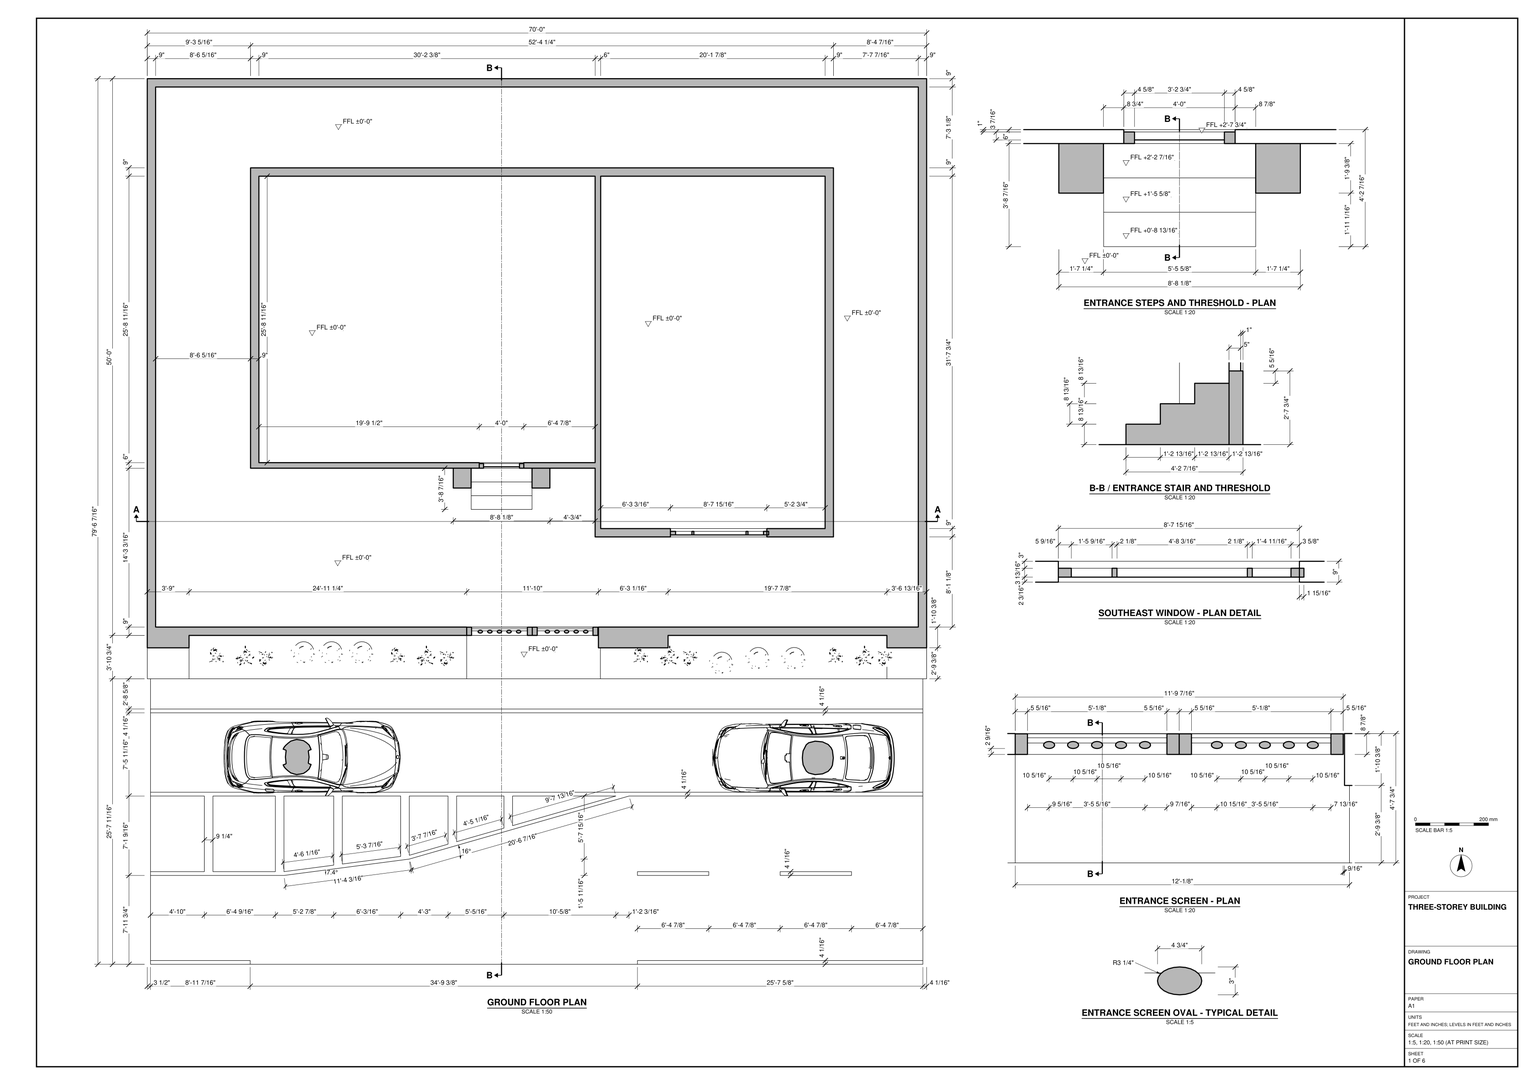
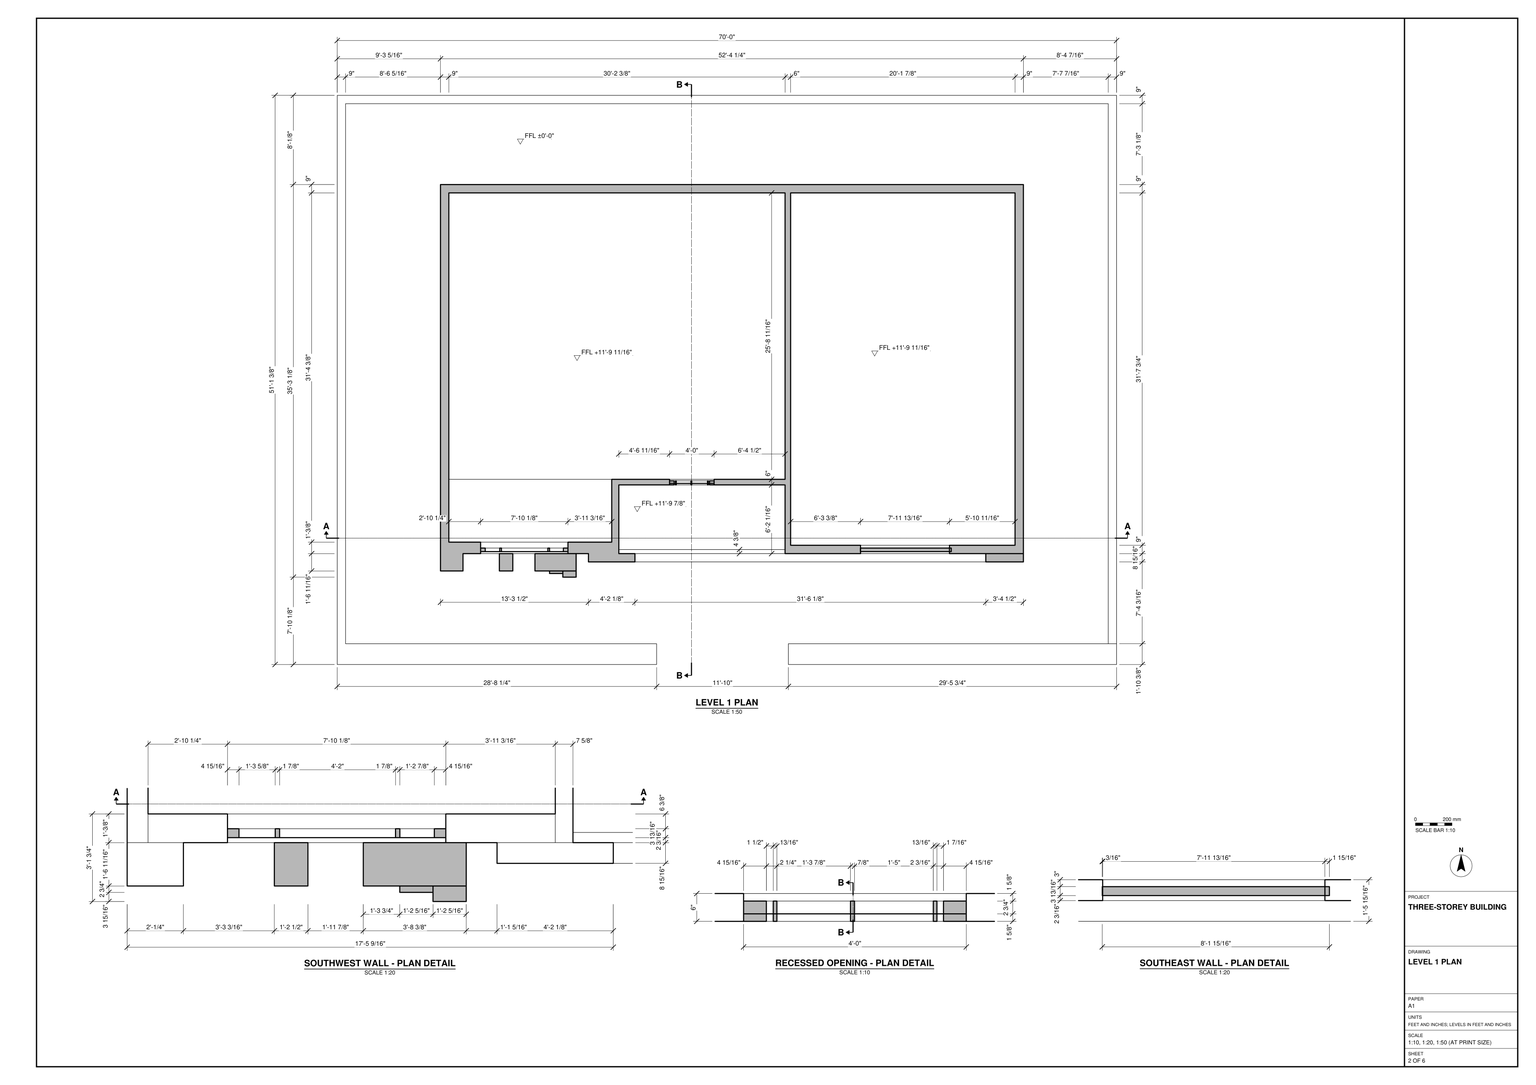
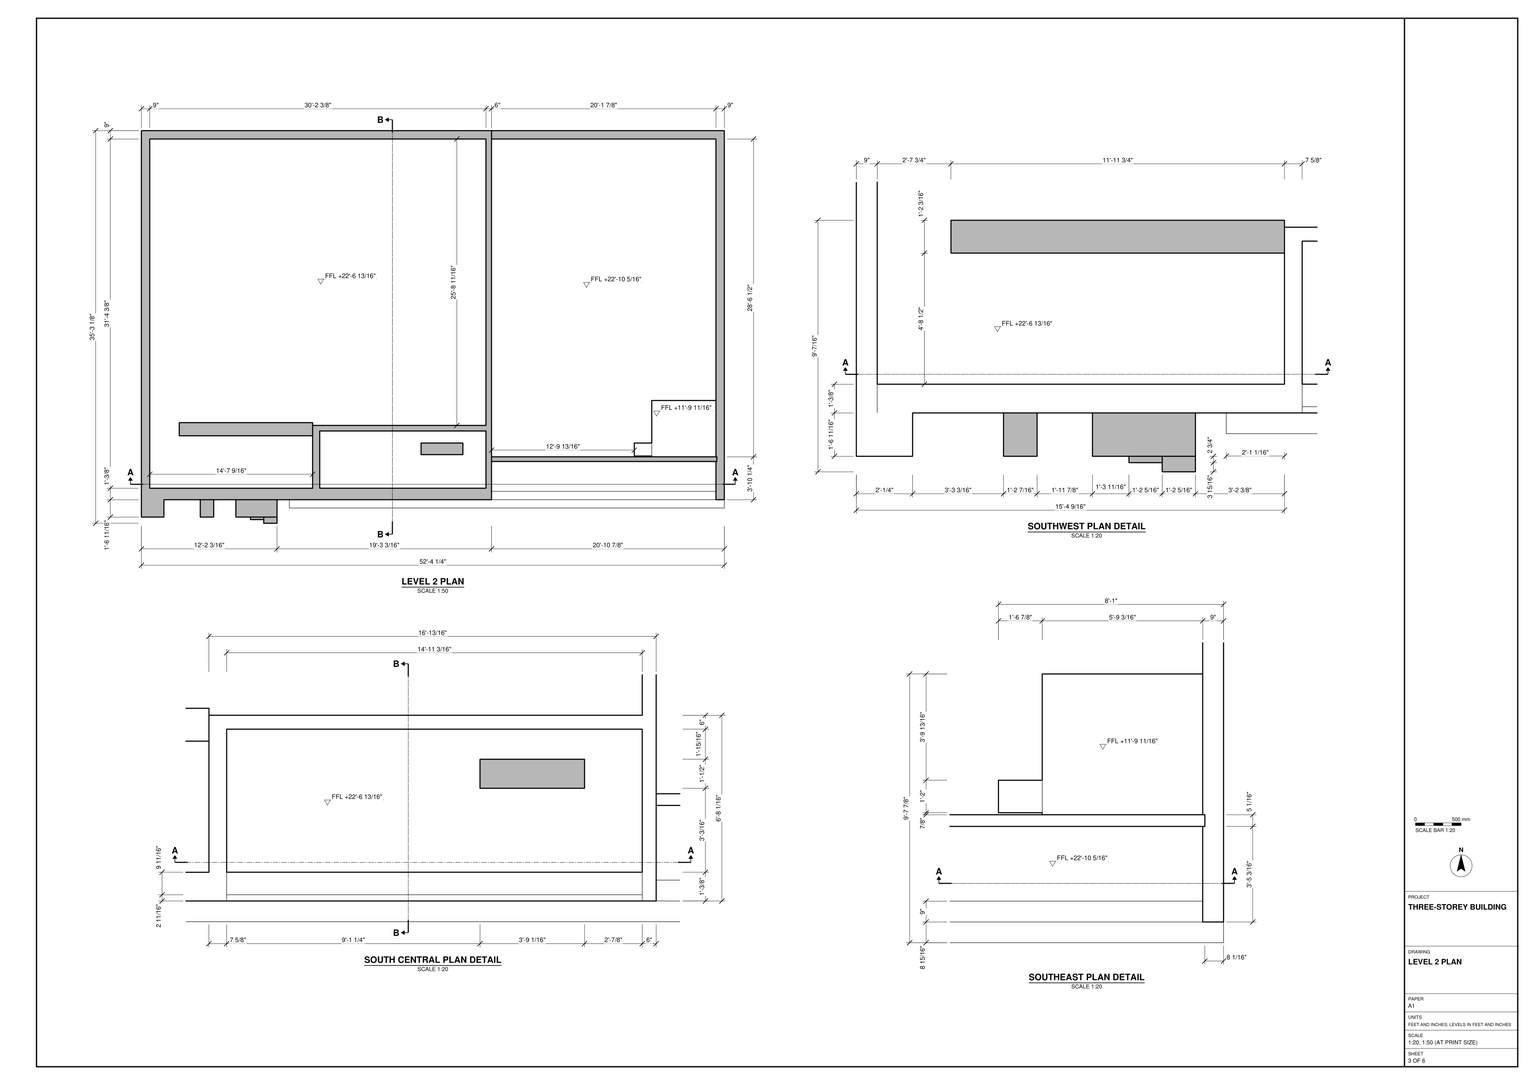
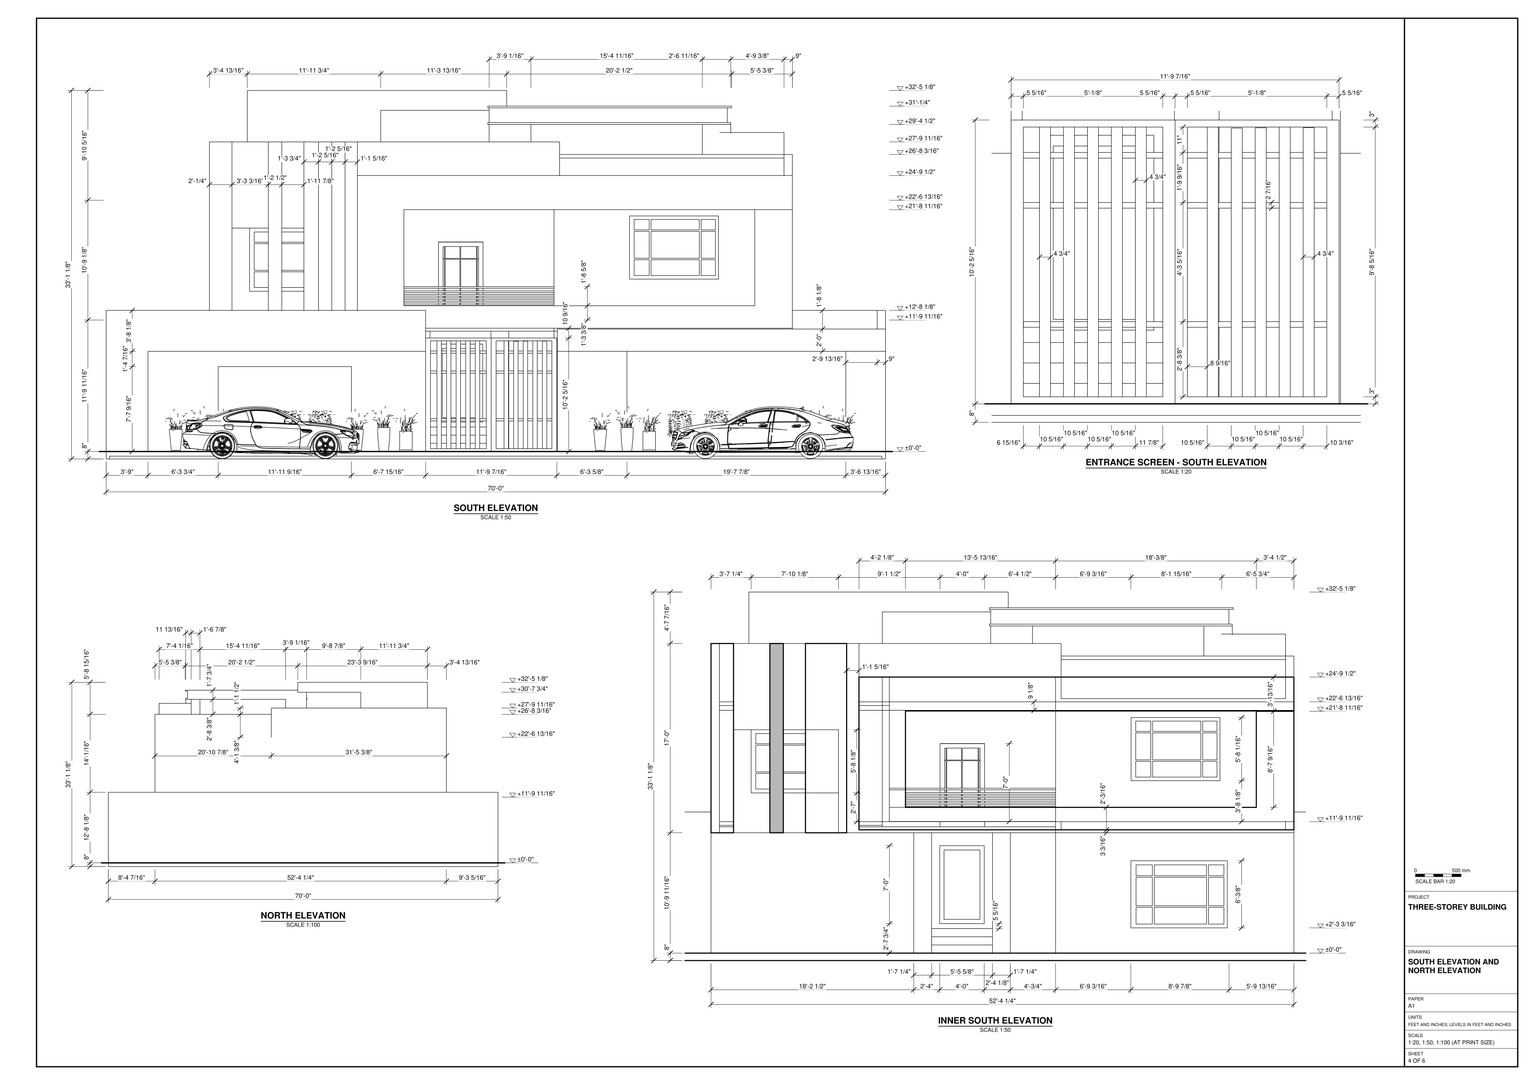
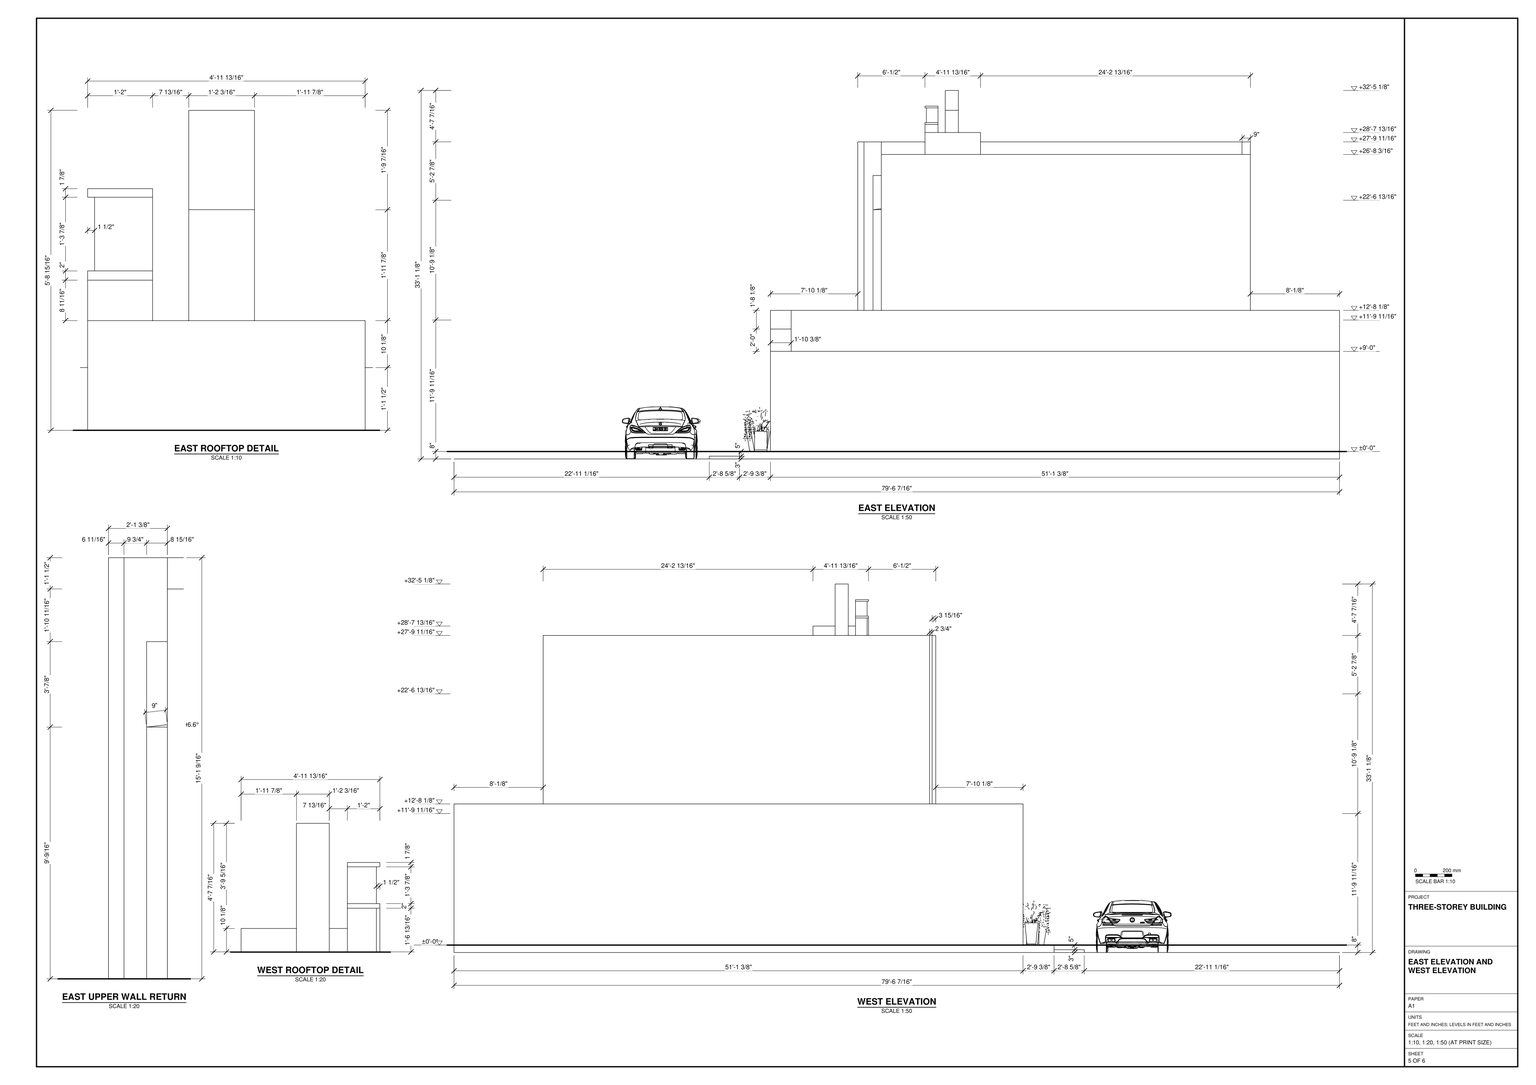
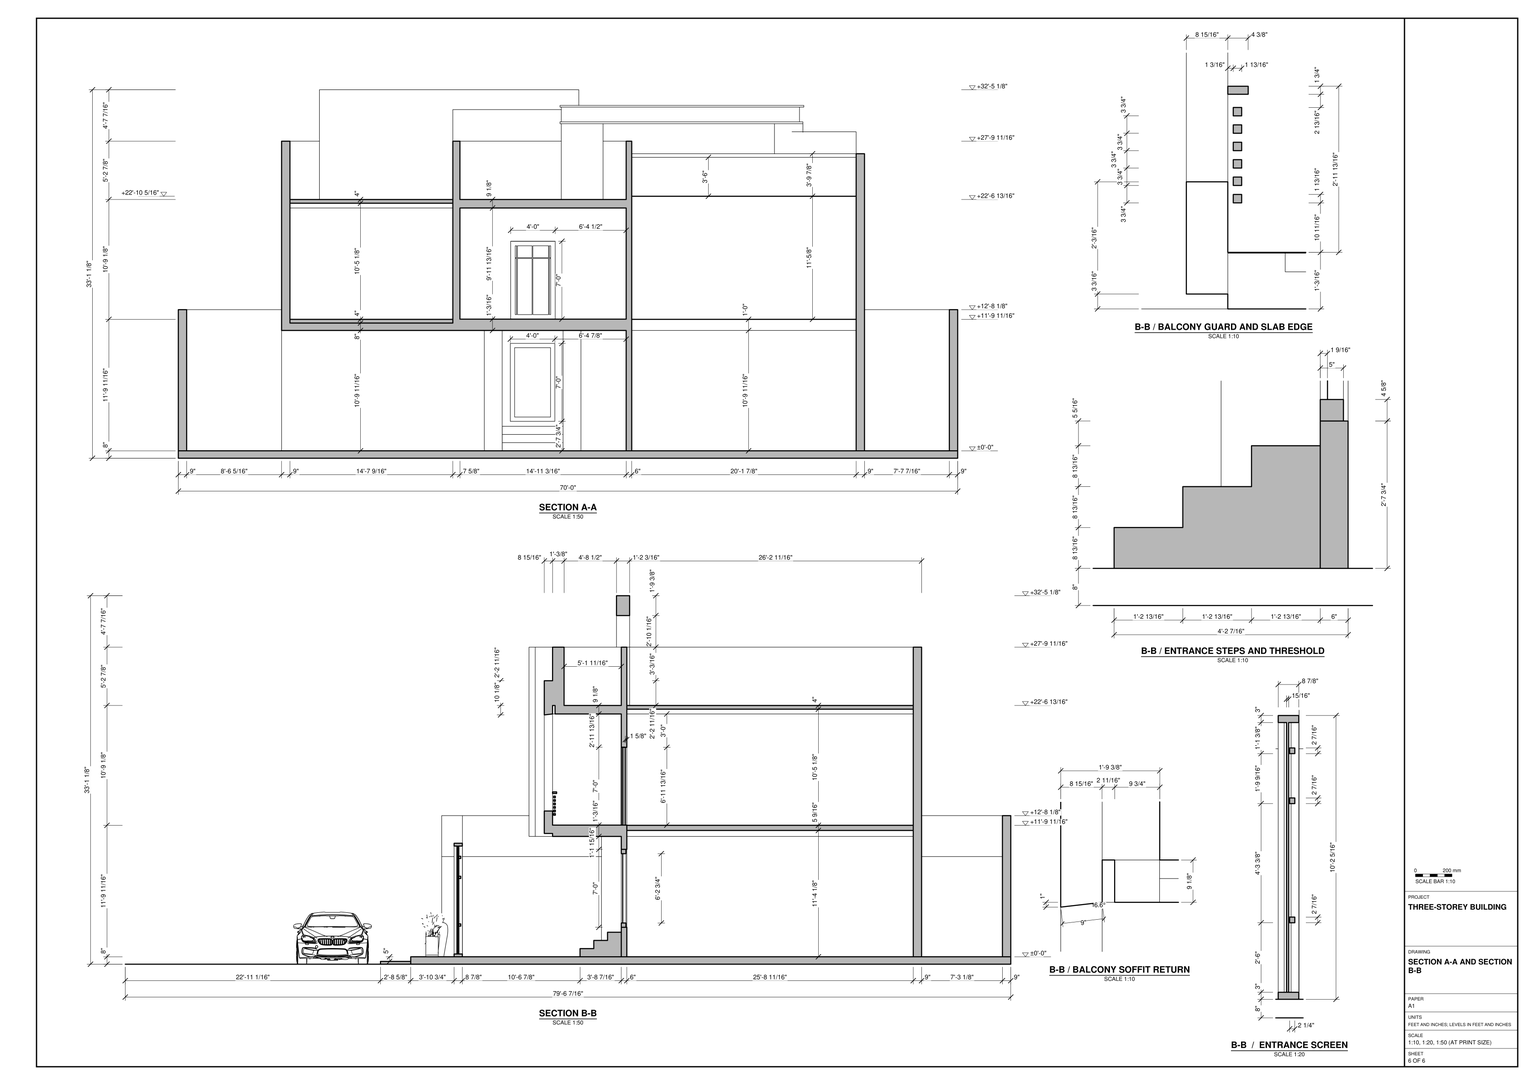
Build the three-storey building and its site in SketchUp from task_files/diagram_01.pdf. Work in feet and inches. Including the street frontage, the model measures 70'-0" across, 79'-6 7/16" from front to back and 33'-1 1/8" high. Set the principal floor levels to ±0'-0", +11'-9 11/16" and +22'-6 13/16". Follow the local changes in floor height shown on the plans.

Set the building back from the south boundary as drawn. Divide the shell into the wider west bay and narrower east bay, using the wall thicknesses shown. At ground level, extend the east bay forward of the west entrance wall. Model the entrance steps, threshold and door in the west bay and the framed window in the east bay. Use the upper-floor plans for the recessed central opening, the projecting portions of the southwest wall and the changes in slab outline at the southeast corner. Model the floor slabs and roof to the profiles shown rather than copying the ground-floor footprint upward.

Include the boundary walls, entrance screen, planting strips, two parked cars and street markings in their drawn positions. Planting, vehicles and other loose items may be suitable library components. Keep walls, slabs, roof and any individual furniture or joinery pieces in separate groups or components, and use components for repeated parts. Save one SketchUp model as output_files/three_storey_building_and_its_street_frontage.skp.

# SketchUp Ruby script. Lengths in inches.
U = 1.inch
M = Sketchup.active_model
def pt(a) = Geom::Point3d.new(a.map { |v| v * U })
def face(e, loops, mat)
  f = e.add_face(loops[0].map { |a| pt(a) })
  loops[1..].each { |l| e.add_face(l.map { |a| pt(a) }).erase! }
  f.material = f.back_material = mat if mat
  f
end
# faces: each face lists its corners as indices into pts; further lists are holes
def faces(e, pts, list, mat = nil) = list.each { |f| face(e, (f[0].is_a?(Array) ? f : [f]).map { |l| l.map { |i| pts[i] } }, mat) }
# xy, xz, yz: faces in a plane at the given z, y or x. An outline is a flat list of corners, or four numbers for a rectangle; further outlines are holes
def ring(l) = l.size == 4 ? [[l[0], l[1]], [l[2], l[1]], [l[2], l[3]], [l[0], l[3]]] : l.each_slice(2).to_a
def flat(e, list, mat, &to3) = list.each { |f| face(e, (f[0].is_a?(Array) ? f : [f]).map { |l| ring(l).map { |u, v| to3.(u, v) } }, mat) }
def xy(e, z, list, mat = nil) = flat(e, list, mat) { |x, y| [x, y, z] }
def xz(e, y, list, mat = nil) = flat(e, list, mat) { |x, z| [x, y, z] }
def yz(e, x, list, mat = nil) = flat(e, list, mat) { |y, z| [x, y, z] }
def lines(e, pts, list) = list.each { |a, b| e.add_line(pt(pts[a]), pt(pts[b])) }
# prism: a flat outline (further loops are holes) pulled along v
def prism(e, loops, v, mat = nil)
  f = face(e, loops, mat); d = Geom::Vector3d.new(v.map { |x| x * U })
  f.pushpull(f.normal.samedirection?(d) ? d.length : -d.length)
end
def box(e, o, s, mat = nil) = prism(e, [[o, [o[0] + s[0], o[1], o[2]], [o[0] + s[0], o[1] + s[1], o[2]], [o[0], o[1] + s[1], o[2]]]], [0, 0, s[2]], mat)
def at(x, y, z, deg = 0) = Geom::Transformation.translation(pt([x, y, z])) * Geom::Transformation.rotation(ORIGIN, Z_AXIS, deg.degrees)
def axes(o, x, y, z) = Geom::Transformation.new([*x, 0, *y, 0, *z, 0, *pt(o).to_a, 1])
def part(name) = M.definitions.add(name)
# library, detail: a bought-in or finely detailed component or shape, given as its bounding box
def library(name, o, s) = part(name).tap { |d| box(d.entities, o, s) }
def detail(e, o, s) = box(e.add_group.entities, o, s)
def put(e, d, t, mat = nil) = e.add_instance(d, t).tap { |i| i.material = mat if mat }
def group(e, t, mat = nil) = e.add_group.tap { |g| g.transformation = t; g.material = mat if mat }.entities
root = M.entities
M.materials.add("[Asphalt New]").color = [67, 60, 62]
M.materials.add("[Asphalt_New]").color = [67, 60, 62]
M.materials.add("[Color C08]").color = [102, 51, 0]
M.materials.add("[Color M00]").color = [255, 255, 255]
M.materials.add("[Color M06]").color = [86, 86, 86]
M.materials.add("[Color M08]").color = [58, 25, 30]
M.materials.add("[Color M09]").color = [74, 0, 0]
M.materials.add("[Color_000]").color = [255, 255, 255]
M.materials.add("[Color_D01]").color = [255, 191, 0]
M.materials.add("[Concrete_Form_4x8]").color = [167, 170, 168]
M.materials.add("[Granite Dark Gray]").color = [69, 68, 68]
M.materials.add("[Stone Vein Gray]").color = [166, 165, 165]
M.materials.add("[Translucent Glass Gray]").color = [128, 128, 128]
M.materials["[Translucent Glass Gray]"].alpha = 0.5
M.materials.add("[Wood Fence]").color = [142, 67, 30]
c1 = library("VASO VIETNAMITA",[-16.09,-10.89,0],[52.51,52.51,44.28])
c2 = part("Road w/ end turnlane")
xy(c2.entities,0,[[359.51,57.5,407.51,596]])
xy(c2.entities,0,[[[-39.49,57.5,-39.49,256.5,-45.49,256.5,-45.49,526.5,-39.49,526.5,-39.49,596,95.51,596,95.51,502.95,121.5,415.58,221.51,262.35,221.51,57.5],[95.51,107.25,101.51,157],[95.51,206.75,101.51,256.5]],[227.51,57.5,353.51,596],[221.51,271.54,174.5,343.5625,221.51,343.5625],[170.59,349.5625,149.04,382.57,221.51,382.57,221.51,349.5625],[145.125,388.57,127.5,415.58,221.51,415.58,221.51,388.57],
  [125.71,421.58,113.61,462.27,221.51,462.27,221.51,421.58],[111.83,468.27,101.51,502.95,221.51,502.95,221.51,468.27],[101.51,508.95,221.51,552.47],[101.51,558.47,221.51,596]],"[Asphalt_New]")
xy(c2.entities,0,[[353.51,57.5,359.51,596],[95.51,107.25,101.51,157],[95.51,206.75,101.51,256.5]],"[Color_000]")
xy(c2.entities,0,[[-45.49,57.5,-39.49,256.5],[[221.51,57.5,221.51,262.35,121.5,415.58,95.51,502.95,95.51,596,101.51,596,101.51,558.47,221.51,558.47,221.51,596,227.51,596,227.51,57.5],[101.51,508.95,221.51,552.47],[125.71,421.58,221.51,421.58,221.51,462.27,113.61,462.27],[111.83,468.27,221.51,468.27,221.51,502.95,101.51,502.95],[145.125,388.57,221.51,388.57,221.51,415.58,127.5,415.58],[170.59,349.5625,221.51,349.5625,221.51,382.57,149.04,382.57],[221.51,271.54,221.51,343.5625,174.5,343.5625]],[-45.49,526.5,-39.49,596]],"[Color_D01]")
xy(c2.entities,3,[[359.51,57.5,407.51,596]],"[Concrete_Form_4x8]")
xz(c2.entities,57.5,[[359.51,0,407.51,3]])
xz(c2.entities,596,[[359.51,0,407.51,3]],"[Concrete_Form_4x8]")
yz(c2.entities,359.51,[[57.5,0,596,3]],"[Concrete_Form_4x8]")
yz(c2.entities,407.51,[[57.5,0,596,3]],"[Concrete_Form_4x8]")
c3 = library("araç",[-7.9,-14.14,0],[84.07,190.26,56.29])
c4 = library("MERCEDES LIGHT",[-74.97,-97.73,0.18],[82.22,195.9,56.22])
c5 = part("Group\#1")
xy(c5.entities,0,[[0,0,100.125,6]],"[Color C08]")
xy(c5.entities,5.27,[[5.27,0,21.9,6],[23.9,0,77.06,6],[79.06,0,94.85,6]],"[Color C08]")
xy(c5.entities,26.63,[[5.27,0,21.9,6],[23.9,0,77.06,6],[79.06,0,94.85,6]],"[Color C08]")
xy(c5.entities,28.63,[[5.27,0,21.9,6],[23.9,0,77.06,6],[79.06,0,94.85,6]],"[Color C08]")
xy(c5.entities,65.04,[[5.27,0,21.9,6],[23.9,0,77.06,6],[79.06,0,94.85,6]],"[Color C08]")
xy(c5.entities,67.04,[[5.27,0,21.9,6],[23.9,0,77.06,6],[79.06,0,94.85,6]],"[Color C08]")
xy(c5.entities,80.98,[[5.27,0,21.9,6],[23.9,0,77.06,6],[79.06,0,94.85,6]],"[Color C08]")
xy(c5.entities,86.25,[[0,0,100.125,6]],"[Color C08]")
xz(c5.entities,0,[[[0,0,100.125,86.25],[23.9,28.63,77.06,65.04],[23.9,5.27,77.06,26.63],[23.9,67.04,77.06,80.98],[5.27,28.63,21.9,65.04],[79.06,28.63,94.85,65.04],[5.27,5.27,21.9,26.63],[79.06,5.27,94.85,26.63],[5.27,67.04,21.9,80.98],[79.06,67.04,94.85,80.98]]],"[Color C08]")
xz(c5.entities,0,[[5.27,5.27,21.9,26.63],[23.9,5.27,77.06,26.63],[79.06,5.27,94.85,26.63],[5.27,28.63,21.9,65.04],[23.9,28.63,77.06,65.04],
  [79.06,28.63,94.85,65.04],[5.27,67.04,21.9,80.98],[23.9,67.04,77.06,80.98],[79.06,67.04,94.85,80.98]],"[Translucent Glass Gray]")
xz(c5.entities,6,[[[0,0,100.125,86.25],[23.9,28.63,77.06,65.04],[23.9,5.27,77.06,26.63],[23.9,67.04,77.06,80.98],[5.27,28.63,21.9,65.04],[79.06,28.63,94.85,65.04],[5.27,5.27,21.9,26.63],[79.06,5.27,94.85,26.63],[5.27,67.04,21.9,80.98],[79.06,67.04,94.85,80.98]]],"[Color C08]")
yz(c5.entities,0,[[0,0,6,86.25]])
yz(c5.entities,5.27,[[0,5.27,6,26.63],[0,28.63,6,65.04],[0,67.04,6,80.98]],"[Color C08]")
yz(c5.entities,21.9,[[0,5.27,6,26.63],[0,28.63,6,65.04],[0,67.04,6,80.98]],"[Color C08]")
yz(c5.entities,23.9,[[0,5.27,6,26.63],[0,28.63,6,65.04],[0,67.04,6,80.98]],"[Color C08]")
yz(c5.entities,77.06,[[0,5.27,6,26.63],[0,28.63,6,65.04],[0,67.04,6,80.98]],"[Color C08]")
yz(c5.entities,79.06,[[0,5.27,6,26.63],[0,28.63,6,65.04],[0,67.04,6,80.98]],"[Color C08]")
yz(c5.entities,94.85,[[0,5.27,6,26.63],[0,28.63,6,65.04],[0,67.04,6,80.98]],"[Color C08]")
yz(c5.entities,100.125,[[0,0,6,86.25]],"[Color C08]")
c6 = library("Group\#2",[0,0,0],[48,4.375,84])
c7 = library("Group\#4",[0,0,0],[88.9375,8.875,134.4375])
c8 = library("Group\#6",[0,0,0],[79.77,27.28,49.07])
xy(root,0,[[0,307.71,840,954.46]])
xy(root,8,[[344.27,307.71,488.375,307.71,488.375,341.09,486.25,341.09,486.25,363.46,344.27,363.46],[0,341.09,0,954.46,840,954.46,840,341.09,797.19,341.09,797.19,354.46,561.29,354.46,561.29,341.09,486.25,341.09,486.25,363.46,831,363.46,831,945.46,9,945.46,9,363.46,344.27,363.46,344.27,354.46,45.03,354.46,45.03,341.09],[[9,363.46,831,945.46],[482.6875,460.59,482.6875,534.65,433.93,534.65,433.93,513.27,414.68,513.27,414.68,490.21,349.12,490.21,349.12,534.65,349.06,534.65,349.06,513.27,329.81,513.27,329.81,534.65,111.3125,534.65,111.3125,858.34,739.5625,858.34,739.5625,460.59]],[[482.6875,460.59,482.6875,534.65,111.3125,534.65,111.3125,858.34,739.5625,858.34,739.5625,460.59],[120.3125,540.65,482.6875,849.34],[488.6875,469.59,730.5625,849.34]],[488.6875,469.59,730.5625,849.34],
  [349.12,490.21,414.68,505.02],[349.12,505.02,414.68,534.65],[120.3125,540.65,482.6875,849.34]])
xy(root,8,[[0,307.71,45.03,341.09],[45.03,307.71,344.27,354.46],[488.375,307.71,797.19,307.71,797.19,354.46,561.29,354.46,561.29,341.09,488.375,341.09],[797.19,307.71,840,341.09]],"[Stone Vein Gray]")
xy(root,16.8125,[[349.12,490.21,414.68,505.02]])
xy(root,25.625,[[349.12,505.02,414.68,519.84]])
xy(root,34.4375,[[349.12,519.84,414.68,534.65]])
xy(root,35.21,[[563.85,460.59,667.79,469.59]])
xy(root,39.77,[[357.8125,534.65,405.8125,540.65]])
xy(root,107.58,[[563.85,460.59,667.79,469.59]])
xy(root,116,[[45.03,341.09,344.27,354.46],[486.25,341.09,486.25,363.46,840,363.46,840,341.09,797.19,341.09,797.19,354.46,561.29,354.46,561.29,341.09],[561.29,341.09,797.19,354.46]])
xy(root,123.77,[[357.8125,534.65,405.8125,540.65]])
xy(root,137.6875,[[243.17,435.21,257.49,441.9],[228.85,439.15,243.17,441.9],[111.3125,441.9,135.57,460.59],[174.77,441.9,189.24,460.59],[213.12,441.9,257.49,460.59],
  [111.3125,460.59,329.81,534.65],[329.81,460.59,349.06,513.27],[349.06,460.59,414.68,534.65],[414.68,460.59,433.93,513.27],[433.93,460.59,482.6875,534.65],
  [329.81,513.27,349.06,534.65],[414.68,513.27,433.93,534.65]])
xy(root,140,[[486.25,341.09,840,363.46]])
xy(root,140.9,[[270.78,451.65,739.5625,460.59]],"[Granite Dark Gray]")
xy(root,144.125,[[120.3125,540.65,482.6875,849.34]])
xy(root,145.6875,[[120.3125,472.96,295.88,540.65]])
xy(root,149.6875,[[488.6875,469.59,730.5625,849.34],[120.3125,472.96,295.88,540.65],[120.3125,540.65,482.6875,849.34]])
xy(root,149.875,[[303.52,460.59,482.6875,460.59,482.6875,534.65,406.22,534.65,406.22,540.65,358.22,540.65,358.22,534.65,303.52,534.65]])
xy(root,160.125,[[0,341.09,344.27,341.09,344.27,363.46,9,363.46,9,945.46,831,945.46,831,363.46,840,363.46,840,954.46,0,954.46]])
xy(root,160.55,[[303.52,461.76,482.6875,463.57]],"[Color M09]")
xy(root,162.36,[[303.52,461.76,482.6875,463.57]],"[Color M09]")
xy(root,164.3,[[303.52,461.76,482.6875,463.57]],"[Color M09]")
xy(root,165.09,[[320.89,451.65,699.04,460.59]],"[Granite Dark Gray]")
xy(root,166.11,[[303.52,461.76,482.6875,463.57]],"[Color M09]")
xy(root,168.05,[[303.52,461.76,482.6875,463.57]],"[Color M09]")
xy(root,169.86,[[303.52,461.76,482.6875,463.57]],"[Color M09]")
xy(root,171.8,[[303.52,461.76,482.6875,463.57]],"[Color M09]")
xy(root,173.61,[[303.52,461.76,482.6875,463.57]],"[Color M09]")
xy(root,175.55,[[303.52,461.76,482.6875,463.57]],"[Color M09]")
xy(root,177.36,[[303.52,461.76,482.6875,463.57]],"[Color M09]")
xy(root,179.3,[[303.5,461.76,482.6875,463.57]],"[Color M09]")
xy(root,180.66,[[154.56,460.59,248.69,472.96]])
xy(root,181.11,[[303.5,461.76,482.6875,463.57]],"[Color M09]")
xy(root,183.95,[[303.52,460.59,482.6875,464.98]],"[Color M09]")
xy(root,185.6875,[[303.52,460.59,482.6875,464.98]],"[Color M09]")
xy(root,193.84,[[564.07,460.59,659.88,469.59]])
xy(root,233.6875,[[358.22,534.65,406.22,540.65]])
xy(root,248.79,[[154.56,460.59,248.69,472.96]])
xy(root,261.9,[[564.07,460.59,659.88,469.59]])
xy(root,268.66,[[699.04,451.65,739.5625,460.59]],"[Granite Dark Gray]")
xy(root,269.6875,[[303.52,463.27,482.6875,534.65]])
xy(root,274.8125,[[120.3125,472.96,120.3125,849.34,482.6875,849.34,482.6875,540.65,295.88,540.65,295.88,472.96]])
xy(root,278.8125,[[303.52,460.59,482.6875,463.27],[120.3125,472.96,295.88,472.96,295.88,529.48,152.11,529.48,152.11,543.65,295.88,543.65,295.88,540.65,482.6875,540.65,482.6875,849.34,120.3125,849.34],[[303.52,472.99,482.6875,534.65],[412.74,509.18,457.81,521.68]]])
xy(root,282.3125,[[488.6875,460.59,730.5625,469.59],[488.6875,469.59,730.5625,501.77],[488.6875,501.77,730.5625,506.82],[730.5625,501.77,731.5,506.82],[488.6875,506.82,661.375,506.82,661.375,567.51,730.5625,567.51,730.5625,849.34,488.6875,849.34],
  [661.375,506.82,730.5625,567.51]])
xy(root,285.09,[[642.52,507.68,661.375,521.68]])
xy(root,305.5,[[270.78,451.65,739.5625,460.59]],"[Granite Dark Gray]")
xy(root,324.29,[[488.6875,501.77,731.5,506.82]])
xy(root,328.17,[[730.5625,460.59,739.5625,460.59,739.5625,858.34,488.6875,858.34,488.6875,849.34,730.5625,849.34,730.5625,506.82,731.5,506.82,731.5,501.77,730.5625,501.77],[488.6875,501.77,731.5,506.82],[661.375,506.82,730.5625,507.68]])
xy(root,341.6875,[[243.17,435.21,257.49,441.9],[228.85,439.15,243.17,441.9],[111.3125,441.9,120.3125,460.59],[120.3125,441.9,135.57,460.59],[174.77,441.9,189.24,460.59],
  [213.12,441.9,257.49,460.59],[[111.3125,460.59,120.3125,460.59,120.3125,849.34,482.6875,849.34,482.6875,540.65,295.88,540.65,295.88,472.96,120.3125,472.96,120.3125,460.59,488.6875,460.59,488.6875,858.34,111.3125,858.34],[303.52,472.99,482.6875,534.65]]])
xy(root,351.8125,[[661.375,507.68,730.5625,567.51]])
xy(root,360.53,[[411.37,507.68,457.81,509.18],[457.81,507.68,642.52,521.68],[642.52,507.68,661.375,521.68],[661.375,507.68,673.1875,521.68],[411.37,509.18,412.74,521.68]])
xy(root,362.53,[[411.37,507.68,501.41,509.18],[501.41,507.68,673.1875,509.18],[411.37,509.18,412.74,521.68],[669.5,509.18,673.1875,521.68]],"[Color M06]")
xy(root,375.72,[[295.88,529.48,431.68,543.65]])
xy(root,378.39,[[411.37,507.68,412.74,521.68],[412.74,507.68,674.1875,509.18],[669.5,509.18,674.1875,521.68]])
xy(root,380.25,[[411.37,507.68,674.1875,521.68]],"[Color M06]")
xy(root,397.125,[[152.11,529.48,431.68,543.65]])
xz(root,307.71,[[0,0,840,8]],"[Stone Vein Gray]")
xz(root,341.09,[[0,8,45.03,8,45.03,116,344.27,116,344.27,160.125,0,160.125],[486.25,8,561.29,116],[797.19,8,840,116],[486.25,116,840,140]])
xz(root,354.46,[[[45.03,8,344.27,116],[120.77,14.29,264.33,99.54]],[561.29,8,797.19,116]])
xz(root,354.46,[[120.77,14.29,264.33,99.54]],"[Asphalt New]")
xz(root,363.46,[[9,8,344.27,160.125],[486.25,8,831,116],[486.25,116,831,140],[831,116,840,140],[831,140,840,160.125]])
xz(root,435.21,[[243.17,137.6875,257.49,341.6875]])
xz(root,439.15,[[228.85,137.6875,243.17,341.6875]])
xz(root,441.9,[[111.3125,137.6875,135.57,341.6875],[174.77,137.6875,189.24,341.6875],[213.12,137.6875,228.85,341.6875],[228.85,137.6875,243.17,341.6875],[243.17,137.6875,257.49,341.6875]])
xz(root,451.65,[[[270.78,140.9,739.5625,305.5],[320.89,165.09,699.04,268.66]]],"[Granite Dark Gray]")
xz(root,460.59,[[[482.6875,8,739.5625,137.6875],[563.85,35.21,667.79,107.58]],[135.57,137.6875,174.77,137.6875,174.77,180.66,154.56,180.66,154.56,248.79,135.57,248.79],[174.77,137.6875,189.24,180.66],[189.24,137.6875,213.12,180.66],[213.12,137.6875,248.69,180.66],
  [248.69,137.6875,257.49,137.6875,257.49,341.6875,213.12,341.6875,213.12,248.79,248.69,248.79],[257.49,137.6875,482.6875,137.6875,482.6875,140.9,270.78,140.9,270.78,341.6875,257.49,341.6875],[482.6875,137.6875,739.5625,140.9],[482.6875,149.6875,739.5625,149.6875,739.5625,268.66,699.04,268.66,699.04,165.09,482.6875,165.09],[303.52,149.875,482.6875,165.09],
  [303.52,165.09,320.89,183.95],[174.77,180.66,189.24,248.79],[213.12,180.66,248.69,248.79],[303.52,183.95,320.89,185.6875],[303.52,185.6875,320.89,269.6875],
  [174.77,248.79,189.24,341.6875],[303.52,269.6875,482.6875,278.8125],[482.6875,269.6875,739.5625,278.8125],[482.6875,278.8125,739.5625,278.8125,739.5625,305.5,730.5625,305.5,730.5625,282.3125,488.6875,282.3125,488.6875,305.5,482.6875,305.5],[270.78,305.5,488.6875,341.6875],
  [730.5625,305.5,739.5625,328.17]])
xz(root,460.59,[[[482.6875,165.09,699.04,165.09,699.04,268.66,739.5625,268.66,739.5625,269.6875,482.6875,269.6875],[564.07,193.84,659.88,261.9]]],"[Color M00]")
xz(root,460.59,[[320.89,183.95,482.6875,185.6875]],"[Color M09]")
xz(root,460.59,[[135.57,248.79,174.77,341.6875],[189.24,248.79,213.12,341.6875],[488.6875,282.3125,730.5625,305.5]],"[Granite Dark Gray]")
xz(root,461.76,[[303.52,160.55,482.6875,162.36]])
xz(root,461.76,[[303.52,164.3,482.6875,166.11],[303.52,168.05,482.6875,169.86],[303.52,171.8,482.6875,173.61],[303.52,175.55,482.6875,177.36],[303.5,179.3,482.6875,181.11]],"[Color M09]")
xz(root,463.27,[[303.52,269.6875,482.6875,278.8125]])
xz(root,463.57,[[303.52,160.55,482.6875,162.36],[303.52,164.3,482.6875,166.11],[303.52,168.05,482.6875,169.86],[303.52,171.8,482.6875,173.61],[303.52,175.55,482.6875,177.36],
  [303.5,179.3,482.6875,181.11]],"[Color M09]")
xz(root,464.98,[[303.52,183.95,482.6875,185.6875]],"[Color M09]")
xz(root,469.59,[[[488.6875,8,730.5625,137.6875],[563.85,35.21,667.79,107.58]],[488.6875,137.6875,730.5625,149.6875],[[488.6875,149.6875,730.5625,278.8125],[564.07,193.84,659.88,261.9]],[488.6875,278.8125,730.5625,282.3125]])
xz(root,472.96,[[120.3125,145.6875,295.88,149.6875],[[120.3125,149.6875,295.88,269.6875],[154.56,180.66,248.69,248.79]],[120.3125,269.6875,295.88,274.8125],[120.3125,274.8125,295.88,278.8125],[120.3125,278.8125,295.88,341.6875]])
xz(root,472.99,[[303.52,278.8125,482.6875,341.6875]])
xz(root,490.21,[[349.12,8,414.68,16.8125]])
xz(root,501.77,[[488.6875,282.3125,730.5625,324.29],[730.5625,282.3125,731.5,324.29],[488.6875,324.29,730.5625,328.17],[730.5625,324.29,731.5,328.17]])
xz(root,505.02,[[349.12,16.8125,414.68,25.625]])
xz(root,506.82,[[488.6875,282.3125,661.375,324.29],[661.375,282.3125,730.5625,324.29],[730.5625,282.3125,731.5,324.29],[488.6875,324.29,661.375,328.17],[661.375,324.29,730.5625,328.17],
  [730.5625,324.29,731.5,328.17]])
xz(root,507.68,[[642.52,285.09,661.375,285.09,661.375,328.17,730.5625,328.17,730.5625,351.8125,673.1875,351.8125,673.1875,360.53,642.52,360.53]])
xz(root,507.68,[[411.37,360.53,673.1875,362.53],[411.37,378.39,674.1875,380.25]],"[Color M06]")
xz(root,509.18,[[412.74,362.53,669.5,378.39]],"[Color M06]")
xz(root,509.18,[[412.74,278.8125,457.81,360.53]],"[Wood Fence]")
xz(root,513.27,[[329.81,8,349.06,137.6875],[414.68,8,433.93,137.6875]])
xz(root,519.84,[[349.12,25.625,414.68,34.4375]])
xz(root,521.68,[[661.375,351.28,673.1875,360.53]],"[Color M06]")
xz(root,521.68,[[412.74,278.8125,412.74,360.53,411.37,360.53,411.37,362.53,412.74,362.53,412.74,378.39,411.37,378.39,411.37,380.25,674.1875,380.25,674.1875,378.39,669.5,378.39,669.5,362.53,673.1875,362.53,673.1875,360.53,457.81,360.53,457.81,278.8125],[642.52,285.09,661.375,360.53]],"[Wood Fence]")
xz(root,529.48,[[152.11,278.8125,295.88,278.8125,295.88,375.72,431.68,375.72,431.68,397.125,152.11,397.125]])
xz(root,534.65,[[111.3125,8,329.81,137.6875],[329.81,8,349.06,137.6875],[[349.06,8,349.12,8,349.12,34.4375,414.68,34.4375,414.68,137.6875,349.06,137.6875],[357.8125,39.77,405.8125,123.77]],[349.12,8,414.68,25.625],[414.68,8,433.93,137.6875],
  [433.93,8,482.6875,137.6875],[349.12,25.625,414.68,34.4375],[303.52,149.875,358.22,149.875,358.22,233.6875,406.22,233.6875,406.22,149.875,482.6875,149.875,482.6875,269.6875,303.52,269.6875],[303.52,278.8125,482.6875,341.6875]])
xz(root,540.65,[[[120.3125,8,482.6875,137.6875],[357.8125,39.77,405.8125,123.77]],[120.3125,137.6875,482.6875,144.125],[120.3125,144.125,295.88,145.6875],[295.88,144.125,358.22,149.6875],[358.22,144.125,406.22,149.6875],
  [406.22,144.125,482.6875,149.6875],[120.3125,145.6875,295.88,149.6875],[295.88,149.6875,295.88,269.6875,482.6875,269.6875,482.6875,149.6875,406.22,149.6875,406.22,233.6875,358.22,233.6875,358.22,149.6875],[358.22,149.6875,406.22,149.875],[295.88,269.6875,482.6875,274.8125],
  [295.88,274.8125,482.6875,278.8125],[295.88,278.8125,482.6875,341.6875]])
xz(root,543.65,[[152.11,278.8125,152.11,397.125,431.68,397.125,431.68,375.72,295.88,375.72,295.88,278.8125]])
xz(root,567.51,[[661.375,282.3125,730.5625,351.8125]])
xz(root,849.34,[[120.3125,8,482.6875,137.6875],[488.6875,8,730.5625,137.6875],[120.3125,137.6875,482.6875,144.125],[488.6875,137.6875,730.5625,149.6875],[120.3125,144.125,482.6875,149.6875],
  [120.3125,149.6875,482.6875,269.6875],[488.6875,149.6875,730.5625,282.3125],[120.3125,269.6875,482.6875,274.8125],[120.3125,274.8125,482.6875,278.8125],[120.3125,278.8125,482.6875,341.6875],
  [488.6875,282.3125,730.5625,328.17]])
xz(root,858.34,[[111.3125,8,111.3125,341.6875,488.6875,341.6875,488.6875,328.17,739.5625,328.17,739.5625,8]])
xz(root,945.46,[[9,8,831,160.125]])
xz(root,954.46,[[0,0,840,8],[0,8,840,160.125]])
yz(root,0,[[307.71,0,954.46,8],[341.09,8,954.46,160.125]])
yz(root,9,[[363.46,8,945.46,116],[363.46,116,945.46,160.125]])
yz(root,45.03,[[341.09,8,354.46,116]])
yz(root,111.3125,[[534.65,8,858.34,137.6875],[441.9,137.6875,858.34,341.6875]])
yz(root,120.3125,[[540.65,8,849.34,137.6875],[540.65,137.6875,849.34,144.125],[540.65,144.125,575.52,149.6875],[575.52,144.125,849.34,149.6875],[472.96,145.6875,540.65,149.6875],
  [472.96,149.6875,849.34,269.6875],[472.96,269.6875,849.34,274.8125],[472.96,274.8125,501.01,278.8125],[501.01,274.8125,510.07,278.8125],[510.07,274.8125,849.34,278.8125],
  [472.96,278.8125,849.34,341.6875]])
yz(root,135.57,[[441.9,137.6875,460.59,341.6875]])
yz(root,152.11,[[529.48,278.8125,543.65,397.125]])
yz(root,154.56,[[460.59,180.66,472.96,248.79]])
yz(root,174.77,[[441.9,137.6875,460.59,341.6875]])
yz(root,189.24,[[441.9,137.6875,460.59,341.6875]])
yz(root,213.12,[[441.9,137.6875,460.59,341.6875]])
yz(root,228.85,[[439.15,137.6875,441.9,341.6875]])
yz(root,243.17,[[435.21,137.6875,439.15,341.6875],[439.15,137.6875,441.9,341.6875]])
yz(root,248.69,[[460.59,180.66,472.96,248.79]])
yz(root,257.49,[[435.21,137.6875,441.9,341.6875],[441.9,137.6875,460.59,341.6875]])
yz(root,270.78,[[451.65,140.9,460.59,305.5]],"[Granite Dark Gray]")
yz(root,295.88,[[472.96,145.6875,540.65,149.6875],[472.96,149.6875,540.65,269.6875],[472.96,269.6875,540.65,274.8125],[472.96,274.8125,540.65,278.8125],[472.96,278.8125,529.48,341.6875],
  [529.48,278.8125,540.65,341.6875],[540.65,278.8125,543.65,341.6875],[529.48,341.6875,543.65,375.72]])
yz(root,303.5,[[461.76,179.3,463.57,181.11]])
yz(root,303.52,[[[460.59,149.875,534.65,149.875,534.65,269.6875,460.59,269.6875,460.59,185.6875,464.98,185.6875,464.98,183.95,460.59,183.95],[461.76,171.8,463.57,173.61],[461.76,168.05,463.57,169.86],[461.76,164.3,463.57,166.11],[461.76,160.55,463.57,162.36],[461.76,175.55,463.57,177.36]],[460.59,269.6875,463.27,278.8125],[472.99,278.8125,534.65,341.6875]])
yz(root,320.89,[[451.65,165.09,460.59,165.09,460.59,269.6875,451.65,268.66]],"[Granite Dark Gray]")
yz(root,329.81,[[513.27,8,534.65,137.6875]])
yz(root,344.27,[[354.46,8,363.46,116],[341.09,116,363.46,160.125]])
yz(root,349.06,[[513.27,8,534.65,137.6875]])
yz(root,349.12,[[490.21,8,490.21,16.8125,505.02,16.8125,505.02,25.625,519.84,25.625,519.84,34.4375,534.65,34.4375,534.65,8]])
yz(root,357.8125,[[534.65,39.77,540.65,123.77]])
yz(root,358.22,[[534.65,149.875,540.65,233.6875]])
yz(root,405.8125,[[534.65,39.77,540.65,123.77]])
yz(root,406.22,[[534.65,149.875,540.65,233.6875]])
yz(root,411.37,[[507.68,360.53,521.68,362.53],[507.68,378.39,521.68,380.25]],"[Color M06]")
yz(root,412.74,[[509.18,278.8125,521.68,360.53]])
yz(root,412.74,[[509.18,362.53,521.68,378.39]],"[Color M06]")
yz(root,414.68,[[490.21,8,513.27,8,513.27,25.625,505.02,25.625,505.02,16.8125,490.21,16.8125],[513.27,8,534.65,8,534.65,34.4375,519.84,34.4375,519.84,25.625,513.27,25.625],[513.27,25.625,513.27,137.6875,534.65,137.6875,534.65,34.4375,519.84,34.4375,519.84,25.625]])
yz(root,431.68,[[529.48,375.72,543.65,397.125]])
yz(root,433.93,[[513.27,8,534.65,137.6875]])
yz(root,457.81,[[509.18,278.8125,521.68,360.53]],"[Wood Fence]")
yz(root,482.6875,[[460.59,8,534.65,137.6875],[540.65,8,849.34,137.6875],[540.65,137.6875,849.34,144.125],[540.65,144.125,849.34,149.6875],[540.65,149.6875,849.34,269.6875],
  [464.98,149.875,464.98,185.6875,460.59,185.6875,460.59,269.6875,534.65,269.6875,534.65,149.875],[461.76,160.55,463.57,162.36],[461.76,175.55,463.57,177.36],[461.76,179.3,463.57,181.11],[460.59,183.95,464.98,185.6875],
  [460.59,269.6875,463.27,278.8125],[540.65,269.6875,849.34,274.8125],[540.65,274.8125,849.34,278.8125],[472.99,278.8125,534.65,341.6875],[540.65,278.8125,849.34,341.6875]])
yz(root,482.6875,[[[460.59,149.875,464.98,183.95],[461.76,179.3,463.57,181.11],[461.76,175.55,463.57,177.36],[461.76,171.8,463.57,173.61],[461.76,168.05,463.57,169.86],[461.76,164.3,463.57,166.11],[461.76,160.55,463.57,162.36]]],"[Color M09]")
yz(root,486.25,[[341.09,8,363.46,116],[341.09,116,363.46,140]])
yz(root,488.6875,[[469.59,8,849.34,137.6875],[469.59,137.6875,849.34,149.6875],[469.59,149.6875,849.34,269.6875],[469.59,269.6875,849.34,278.8125],[469.59,278.8125,849.34,282.3125],
  [849.34,278.8125,858.34,328.17],[460.59,282.3125,501.77,282.3125,501.77,328.17,506.82,328.17,506.82,282.3125,849.34,282.3125,849.34,341.6875,460.59,341.6875],[501.77,324.29,506.82,328.17],[849.34,328.17,858.34,341.6875]])
yz(root,561.29,[[341.09,8,354.46,116]])
yz(root,563.85,[[460.59,35.21,469.59,107.58]])
yz(root,564.07,[[460.59,193.84,469.59,261.9]])
yz(root,642.52,[[507.68,285.09,521.68,360.53]],"[Color M06]")
yz(root,659.88,[[460.59,193.84,469.59,261.9]])
yz(root,661.375,[[506.82,282.3125,506.82,328.17,507.68,328.17,507.68,285.09,521.68,285.09,521.68,351.8125,567.51,351.8125,567.51,282.3125]])
yz(root,667.79,[[460.59,35.21,469.59,107.58]])
yz(root,669.5,[[509.18,362.53,521.68,378.39]],"[Color M06]")
yz(root,673.1875,[[507.68,351.28,521.68,360.53],[507.68,360.53,521.68,362.53]],"[Color M06]")
yz(root,674.1875,[[507.68,378.39,521.68,380.25]],"[Color M06]")
yz(root,699.04,[[451.65,165.09,460.59,268.66]],"[Granite Dark Gray]")
yz(root,730.5625,[[469.59,8,849.34,137.6875],[469.59,137.6875,849.34,149.6875],[469.59,149.6875,849.34,282.3125],[460.59,282.3125,469.59,328.17],[469.59,282.3125,501.77,328.17],
  [506.82,282.3125,567.51,328.17],[567.51,282.3125,849.34,328.17],[507.68,328.17,567.51,351.8125]])
yz(root,731.5,[[501.77,282.3125,506.82,324.29],[501.77,324.29,506.82,328.17]])
yz(root,739.5625,[[460.59,8,858.34,328.17]])
yz(root,739.5625,[[451.65,140.9,460.59,268.66],[451.65,268.66,460.59,269.6875,460.59,305.5,451.65,305.5]],"[Granite Dark Gray]")
yz(root,797.19,[[341.09,8,354.46,116]])
yz(root,831,[[363.46,8,945.46,160.125]])
yz(root,840,[[307.71,0,954.46,8],[341.09,8,954.46,116],[341.09,116,363.46,140],[363.46,116,954.46,160.125]])
p = [[482.6875,460.59,269.6875],[711.96,460.59,269.6875],[711.96,451.65,268.66],[699.04,451.65,268.66],[320.89,451.65,268.66],[320.89,460.59,269.6875],
  [739.5625,451.65,268.66],[739.5625,460.59,269.6875],[349.12,519.84,16.8125],[414.68,519.84,16.8125],[120.3125,460.59,269.6875],[120.3125,472.96,269.6875],
  [295.88,472.96,149.6875],[295.88,460.59,149.6875],[120.3125,472.96,149.6875],[120.3125,460.59,149.6875],[488.6875,849.34,269.6875],[488.6875,858.34,269.6875],
  [120.3125,460.59,305.6875],[120.3125,472.96,305.6875],[488.6875,469.59,278.8125],[488.6875,460.59,278.8125],[120.3125,460.59,278.8125],[120.3125,472.96,278.8125],
  [661.375,507.68,351.28],[661.375,521.68,351.28]]
faces(root,p,[[0,1,2,3,4,5],[6,2,1,7]],"[Granite Dark Gray]")
lines(root,p,[[8,9],[10,11],[12,13],[14,15],[16,17],[18,19],[20,21],[22,23],[24,25]])
put(root,c1,at(606.62,307.36,8))
put(root,c1,at(645.8,312.38,8))
put(root,c1,at(155.8125,318.6,8))
put(root,c1,at(186,318.6,8))
put(root,c1,at(218.6875,318.6,8))
put(root,c1,at(684.55,312.38,8))
put(root,c2,axes([924.8125,30.9,0],[0,0.67927,0],[-1.54584,0,0],[0,0,1]))
put(root,c3,at(258.71,189.26,0,90))
put(root,c4,at(707.5625,256.33,-0.18,90))
put(root,c5,axes([154.56,462.75,180.66],[0.94007,0,0],[0,0.64,0],[0,0,0.78986]))
put(root,c5,axes([563.88,462.75,193.47],[0.97815,0,0],[0,0.64,0],[0,0,0.79775]),"[Color M08]")
put(root,c5,axes([563.85,462.75,34.84],[1.05748,0,0],[0,0.64,0],[0,0,0.84338]))
put(root,c6,at(358.22,534.65,149.875))
g1 = group(root,at(357.8125,534.65,39.77))
xy(g1,0,[[0,0,48,5]],"[Color M08]")
xy(g1,4.63,[[4.63,0,43.37,1.5625],[4.63,1.5625,43.37,5]],"[Color M08]")
xy(g1,79.37,[[4.63,0,43.37,1.5625],[4.63,1.5625,43.37,5]],"[Color M08]")
xy(g1,84,[[0,0,48,5]],"[Color M08]")
xz(g1,0,[[[0,0,48,84],[4.63,4.63,43.37,79.37]]],"[Color M08]")
xz(g1,1.5625,[[4.63,4.63,43.37,79.37]],"[Color M08]")
xz(g1,5,[[[0,0,48,84],[4.63,4.63,43.37,79.37]]],"[Color M08]")
yz(g1,0,[[0,0,5,84]],"[Color M08]")
yz(g1,4.63,[[0,4.63,1.5625,79.37],[1.5625,4.63,5,79.37]],"[Color M08]")
yz(g1,43.37,[[0,4.63,1.5625,79.37],[1.5625,4.63,5,79.37]],"[Color M08]")
yz(g1,48,[[0,0,5,84]],"[Color M08]")
put(root,c7,axes([485.68,363.34,8],[-1.59,0,0],[0,-1,0],[0,0,0.91]))
put(root,c8,at(61.34,317.65,8))
put(root,c8,at(256.53,317.65,8))
put(root,c8,at(518.71,317.65,8))
put(root,c8,at(728.72,317.65,8))
